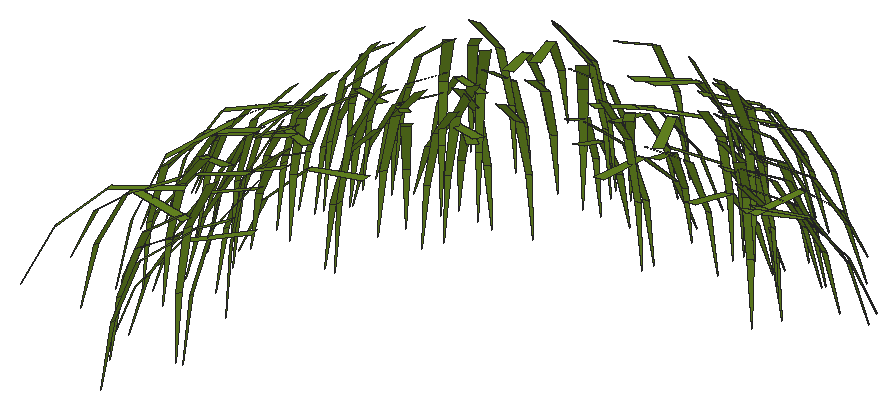
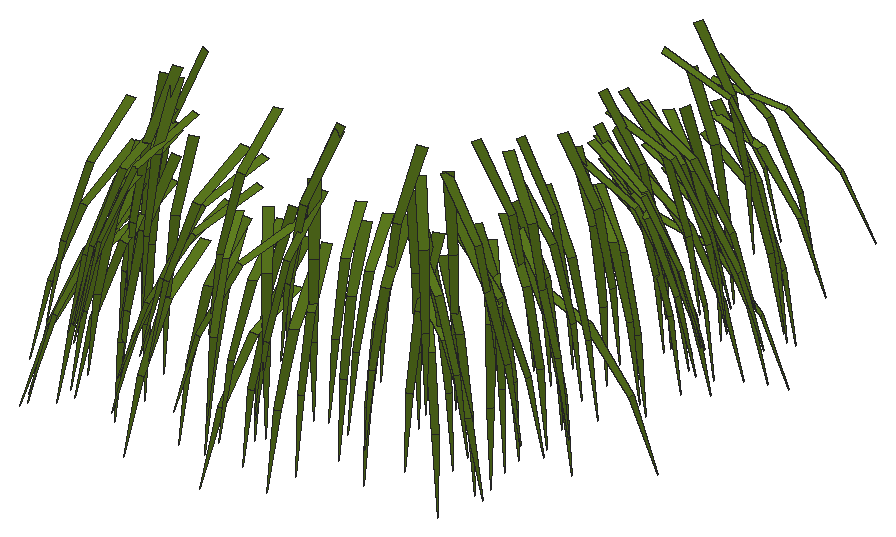
# SketchUp Ruby script. Lengths in inches.
U = 1.inch
M = Sketchup.active_model
def pt(a) = Geom::Point3d.new(a.map { |v| v * U })
def face(e, loops, mat)
  f = e.add_face(loops[0].map { |a| pt(a) })
  loops[1..].each { |l| e.add_face(l.map { |a| pt(a) }).erase! }
  f.material = f.back_material = mat if mat
  f
end
# faces: each face lists its corners as indices into pts; further lists are holes
def faces(e, pts, list, mat = nil) = list.each { |f| face(e, (f[0].is_a?(Array) ? f : [f]).map { |l| l.map { |i| pts[i] } }, mat) }
# xy, xz, yz: faces in a plane at the given z, y or x. An outline is a flat list of corners, or four numbers for a rectangle; further outlines are holes
def ring(l) = l.size == 4 ? [[l[0], l[1]], [l[2], l[1]], [l[2], l[3]], [l[0], l[3]]] : l.each_slice(2).to_a
def flat(e, list, mat, &to3) = list.each { |f| face(e, (f[0].is_a?(Array) ? f : [f]).map { |l| ring(l).map { |u, v| to3.(u, v) } }, mat) }
def xy(e, z, list, mat = nil) = flat(e, list, mat) { |x, y| [x, y, z] }
def xz(e, y, list, mat = nil) = flat(e, list, mat) { |x, z| [x, y, z] }
def yz(e, x, list, mat = nil) = flat(e, list, mat) { |y, z| [x, y, z] }
def lines(e, pts, list) = list.each { |a, b| e.add_line(pt(pts[a]), pt(pts[b])) }
# prism: a flat outline (further loops are holes) pulled along v
def prism(e, loops, v, mat = nil)
  f = face(e, loops, mat); d = Geom::Vector3d.new(v.map { |x| x * U })
  f.pushpull(f.normal.samedirection?(d) ? d.length : -d.length)
end
def box(e, o, s, mat = nil) = prism(e, [[o, [o[0] + s[0], o[1], o[2]], [o[0] + s[0], o[1] + s[1], o[2]], [o[0], o[1] + s[1], o[2]]]], [0, 0, s[2]], mat)
def at(x, y, z, deg = 0) = Geom::Transformation.translation(pt([x, y, z])) * Geom::Transformation.rotation(ORIGIN, Z_AXIS, deg.degrees)
def axes(o, x, y, z) = Geom::Transformation.new([*x, 0, *y, 0, *z, 0, *pt(o).to_a, 1])
def part(name) = M.definitions.add(name)
# library, detail: a bought-in or finely detailed component or shape, given as its bounding box
def library(name, o, s) = part(name).tap { |d| box(d.entities, o, s) }
def detail(e, o, s) = box(e.add_group.entities, o, s)
def put(e, d, t, mat = nil) = e.add_instance(d, t).tap { |i| i.material = mat if mat }
def group(e, t, mat = nil) = e.add_group.tap { |g| g.transformation = t; g.material = mat if mat }.entities
root = M.entities
M.materials.add("[0061_OliveDrab]").color = [107, 142, 35]
p = [[547.6,21.32,549.34],[547.56,21.51,549.34],[547.28,21.36,546.73],[547.37,28.64,549.33],[547.44,28.8125,549.33],[546.91,28.93,546.76],
  [548.89,31.45,549.33],[548.99,31.6,549.33],[548.51,31.82,546.76],[560.32,34.67,549.36],[560.5,34.73,549.36],[560.25,35.21,546.79],
  [546.9,18.21,549.5],[546.87,18.44,549.5],[546.46,18.28,546.91],[545.88,20.63,549.3125],[545.83,20.82,549.3125],[544.94,20.49,546.86],
  [548.84,33.23,549.46],[548.99,33.375,549.46],[548.21,34.05,547.05],[560.09,33.66,549.64],[560.29,33.77,549.64],[560.08,33.92,547.03],
  [555.03,34.76,549.55],[555.24,34.77,549.55],[555.11,35.23,546.97],[558.47,35.98,549.375],[558.68,36.02,549.375],[558.39,37.07,546.98],
  [545.65,27.41,549.44],[545.67,27.625,549.44],[544.48,27.64,547.1],[551.32,33.5,549.6875],[551.51,33.57,549.6875],[551.25,33.95,547.1],
  [562.55,35.57,549.5625],[562.74,35.53,549.5625],[562.83,36.35,547.07],[546.13,20.92,549.68],[546.16,21.11,549.68],[545.27,21.13,547.21],
  [548.18,31.25,549.77],[548.35,31.39,549.77],[547.83,31.85,547.24],[557.26,35.12,549.75],[557.48,35.13,549.75],[557.32,35.67,547.18],
  [553.46,35.38,549.62],[553.67,35.45,549.62],[553.23,36.33,547.18],[562.35,35.82,549.6],[562.54,35.77,549.6],[562.73,36.85,547.21],
  [555,36.3,549.5625],[555.22,36.32,549.5625],[554.97,37.54,547.25],[549.66,31.51,549.93],[549.78,31.7,549.93],[549.43,31.78,547.33],
  [555.36,33.95,549.95],[555.56,33.98,549.95],[555.43,34.2,547.34],[561.75,35.34,549.78],[561.95,35.32,549.78],[561.92,36.05,547.26],
  [546.66,18.8,550.07],[546.73,18.97,550.07],[546.16,19.1,547.51],[548,20.1,550.12],[548.07,20.31,550.12],[547.86,20.26,547.5],
  [548.34,27.75,550.12],[548.36,27.96,550.12],[548.18,27.86,547.5],[550.37,32.6,550.1],[550.58,32.68,550.1],[550.33,33.06,547.52],
  [548.21,30.1,550.19],[548.3125,30.3,550.19],[547.88,30.39,547.6],[556.09,35.37,550.07],[556.27,35.46,550.07],[555.81,36.22,547.6],
  [548.1,32.47,549.99],[548.21,32.67,549.99],[547.11,33.17,547.66],[552.88,34.93,550.2],[553.05,35.01,550.2],[552.64,35.65,547.6875],
  [546.86,23.9375,550.36],[546.91,24.12,550.36],[546.35,24.15,547.79],[560.23,34.5,550.43],[560.44,34.51,550.43],[560.32,34.91,547.84],
  [560.85,35.47,550.33],[561.07,35.45,550.33],[561.04,36.24,547.82],[559.19,35.45,550.33],[559.375,35.4,550.33],[559.49,36.29,547.86],
  [545.93,22.43,550.5],[545.95,22.625,550.5],[545.05,22.65,548.04],[546.07,23.74,550.53],[546.1,23.96,550.53],[545.32,23.95,548.02],
  [561.21,35.4,550.5],[561.41,35.41,550.5],[561.27,36.15,547.98],[546.59,19.18,550.625],[546.67,19.39,550.625],[545.9,19.57,548.12],
  [547.7,31.3,550.62],[547.84,31.43,550.62],[547.17,32,548.14],[548.21,22.54,550.78],[548.16,22.73,550.78],[548.02,22.6,548.16],
  [546.58,25.91,550.64],[546.7,26.1,550.64],[545.9,26.48,548.17],[547.51,30.27,550.71],[547.5625,30.46,550.71],[546.74,30.58,548.21],
  [547.32,29.86,550.89],[547.43,30.03,550.89],[546.82,30.29,548.34],[550.74,31.72,551.06],[550.88,31.86,551.06],[550.67,31.93,548.44],
  [551.68,34.29,550.9],[551.87,34.39,550.9],[551.45,34.98,548.375],[561.55,36.47,550.69],[561.74,36.47,550.69],[561.61,37.81,548.4375],
  [561.05,33.64,551.18],[561.24,33.6,551.18],[561.1875,33.81,548.56],[554.27,34.91,551.1],[554.4375,35.04,551.1],[553.8,35.7,548.64],
  [562.6,35.41,551.08],[562.8,35.375,551.08],[562.84,36.22,548.59],[555.01,35.76,551.05],[555.21,35.82,551.05],[554.83,36.76,548.62],
  [550.99,33.71,551.21],[551.21,33.78,551.21],[550.9,34.34,548.66],[558.8125,34.22,551.34],[559,34.29,551.34],[558.79,34.58,548.74],
  [560.8,35.24,551.18],[561,35.3,551.18],[560.68,36.02,548.67],[546.84,28.06,551.31],[546.9375,28.23,551.31],[546.22,28.51,548.79],
  [553.33,33.7,551.4],[553.51,33.84,551.4],[553.17,34.08,548.81],[546.39,24.22,551.49],[546.43,24.43,551.49],[545.82,24.43,548.9375],
  [547.5625,26.37,551.49],[547.6875,26.56,551.49],[547.31,26.67,548.89],[550.07,30.69,551.52],[550.21,30.83,551.52],[550.02,30.88,548.9],
  [547.75,30.94,551.375],[547.85,31.15,551.375],[546.97,31.42,548.91],[556.42,35.71,551.41],[556.63,35.65,551.41],[556.79,36.55,548.94],
  [545.75,21.83,551.43],[545.77,22.05,551.43],[544.73,22.04,549.02],[547.44,23.9375,551.61],[547.46,24.15,551.61],[547.125,24.08,549],
  [546.24,26.71,551.5625],[546.35,26.875,551.5625],[545.46,27.35,549.14],[547.48,28.04,551.6875],[547.52,28.24,551.6875],[547.08,28.22,549.1],
  [546.59,29.89,551.56],[546.6875,30.05,551.56],[545.8125,30.48,549.125],[554.3,34.92,551.6],[554.49,34.9375,551.6],[554.33,35.5625,549.06],
  [547.46,20.26,551.78],[547.5625,20.45,551.78],[547.14,20.54,549.1875],[548.38,32.75,551.55],[548.49,32.91,551.55],[547.5,33.45,549.18],
  [547.48,21,551.36],[547.41,21.26,551.36],[548.3,21.41,551.87],[548.25,21.68,551.87],[546.69,24.09,551.82],[546.63,24.29,551.82],
  [546.04,24.01,549.27],[545.98,24.67,551.7],[546.03,24.86,551.7],[545.07,25.02,549.26],[548.32,28.2,551.74],[548.42,28.44,551.74],
  [549.72,30.83,551.74],[549.87,31.04,551.74],[555.6875,35.79,551.66],[555.87,35.89,551.66],[555.1875,36.9,549.34],[547.51,25.99,552.04],
  [547.5625,26.2,552.04],[547.2,26.18,549.44],[547.5,27.18,551.28],[547.54,27.48,551.28],[560.59,33.65,551.77],[560.84,33.73,551.77],
  [558.73,34.25,551.33],[559.03,34.3,551.33],[561.19,35.1,551.95],[561.4,35.04,551.95],[561.47,35.73,549.41],[547.86,18.27,551.94],
  [547.82,18.59,551.94],[549.98,31.97,551.46],[550.19,32.17,551.46],[558.5,35.71,551.85],[558.68,35.64,551.85],[558.97,36.68,549.45],
  [560.34,33.11,552.2],[560.62,33.26,552.2],[555.03,33.75,551.98],[555.33,33.77,551.98],[553.96,33.85,551.69],[554.26,33.96,551.69],
  [561.87,34.18,551.59],[562.15,34.11,551.59],[562.18,34.14,551.74],[562.44,34.08,551.74],[555.17,34.36,551.33],[555.48,34.4,551.33],
  [546.45,17.94,552.27],[546.46,18.15,552.27],[545.81,18.09,549.73],[547.59,20.7,551.85],[547.625,20.97,551.85],[548.13,27.53,552.33],
  [548.17,27.7,552.33],[547.89,27.67,549.72],[548.58,30.61,552.29],[548.66,30.79,552.29],[548.1875,30.87,549.71],[551.65,32.57,552.125],
  [551.91,32.67,552.125],[557.3125,33.97,552.11],[557.625,34,552.11],[548.96,30.2,552.05],[549.2,30.4,552.05],[561.59,34.02,552.05],
  [561.875,34,552.05],[546.2,22.5,552.28],[546.3125,22.6875,552.28],[545.34,23.14,549.88],[547.67,23.49,552.53],[547.69,23.6875,552.53],
  [547.37,23.625,549.93],[550.29,31.0625,552.44],[550.46,31.33,552.44],[560.59,33.16,552.49],[560.8,33.23,552.49],[560.625,33.39,549.87],
  [549.6875,31.5,551.84],[549.85,31.78,551.84],[549.71,32.625,552.51],[549.87,32.77,552.51],[549.39,33.15,549.96],[555.42,33.33,552.5],
  [555.69,33.375,552.5],[550.83,34.73,552.36],[551.02,34.82,552.36],[550.49,35.72,549.95],[561.19,35.39,552.49],[561.41,35.35,552.49],
  [561.42,36.11,549.97],[547.75,18.34,552.41],[547.84,18.58,552.41],[548.48,19.9,552.7],[548.58,20.19,552.7],[548.82,27.67,552.7],
  [548.84,27.97,552.7],[548.66,28.85,552.67],[548.7,29.04,552.67],[548.375,29.01,550.07],[550.65,31.7,552.55],[550.9375,31.8,552.55],
  [556.7,33.94,552.18],[556.96,34.0625,552.18],[545.27,19.38,552.45],[545.32,19.57,552.45],[544.02,19.8,550.17],[546.21,22.79,552.67],
  [546.28,22.99,552.67],[545.34,23.22,550.23],[546.9,22.94,552.76],[546.95,23.15,552.76],[546.42,23.15,550.1875],[547.61,29.26,552.79],
  [547.72,29.44,552.79],[547.19,29.63,550.22],[549.02,29.64,552.65],[549.16,29.93,552.65],[551.55,32.36,552.77],[551.75,32.41,552.77],
  [551.57,32.72,550.17],[554.84,32.98,552.83],[555.06,32.96,552.83],[554.97,33.2,550.21],[554.68,33.38,552.85],[554.88,33.375,552.85],
  [554.79,33.68,550.24],[553.46,33.65,552.42],[553.7,33.77,552.42],[558.81,34.03,552.51],[559.06,33.97,552.51],[560.66,34.09,552.55],
  [560.97,34.05,552.55],[551.37,35.08,552.78],[551.55,35.17,552.78],[551.01,35.99,550.35],[562.01,35.45,552.75],[562.2,35.46,552.75],
  [562.03,36.375,550.29],[547.65,19.08,552.98],[547.71,19.26,552.98],[547.32,19.29,550.39],[545.89,22.03,552.87],[545.9,22.25,552.87],
  [544.9,22.2,550.44],[547.9,23.65,552.75],[547.96,23.91,552.75],[545.86,24.75,552.8],[545.91,24.93,552.8],[544.82,25.1,550.42],
  [545.76,24.79,552.77],[545.79,24.97,552.77],[544.67,25.0625,550.39],[560.24,33.62,552.9],[560.53,33.63,552.9],[547.46,22.17,552.62],
  [547.5,22.44,552.62],[547.49,23.51,552.72],[547.53,23.82,552.72],[559.83,34,553.0625],[560.02,34.06,553.0625],[559.79,34.42,550.47],
  [561.24,34.05,552.75],[561.52,34.0625,552.75],[560.78,35.23,553.03],[560.96,35.18,553.03],[561.06,35.89,550.51],[560.89,35.44,552.96],
  [561.09,35.43,552.96],[561.05,36.27,550.48],[557.9,35.66,552.92],[558.11,35.61,552.92],[558.23,36.5,550.45],[557.68,35.7,552.93],
  [557.9,35.7,552.93],[557.79,36.58,550.46],[545.57,16.99,553],[545.52,17.17,553],[544.42,16.77,550.65],[547.4,18.6,553.18],
  [547.3,18.8,553.18],[546.9,18.47,550.6],[547.82,18.66,552.89],[547.93,18.95,552.89],[546.16,22.8,553.14],[546.14,23,553.14],
  [545.4,22.85,550.625],[547.8125,25.07,552.8],[547.98,25.34,552.8],[548.74,30.16,552.74],[548.93,30.35,552.74],[560.5625,33.78,553.16],
  [560.78,33.8,553.16],[560.63,34.14,550.56],[548.88,29.87,552.91],[548.95,30.13,552.91],[560.86,32.22,553.27],[561.04,32.14,553.27],
  [561.01,32.33,550.65],[561.58,34.43,552.35],[561.83,34.4375,552.35],[548.67,22.62,553.36],[548.61,22.875,553.36],[548.36,29.17,553.2],
  [548.5,29.41,553.2],[552.22,33.125,553.1875],[552.49,33.26,553.1875],[555.42,34.14,553.07],[555.7,34.22,553.07],[551.09,31.31,553.63],
  [551.29,31.5,553.63],[555.2,33.64,553.2],[555.44,33.82,553.2],[562.33,34.01,553.29],[562.62,33.97,553.29],[551.34,32.54,553.53],
  [551.64,32.64,553.53],[560.9,33.13,553.75],[561.17,33.08,553.75],[561.13,33.91,553.41],[561.41,33.99,553.41],[550.03,26.88,551.92],
  [550.07,27.25,551.92],[547.99,27.38,553.57],[548.12,27.625,553.57],[555.43,31.79,551.8],[555.81,31.84,551.8],[559.12,31.8,552.18],
  [559.49,31.86,552.18],[559.06,33.42,553.83],[559.33,33.53,553.83],[549.88,21.58,552.25],[549.8,21.9,552.25],[547.41,21.63,553.46],
  [547.44,21.93,553.46],[549.08,30.29,553.55],[549.21,30.57,553.55],[553.85,32.97,553.87],[554.09,33.17,553.87],[555.92,34.18,553.48],
  [556.21,34.09,553.48],[556.33,34.71,553.93],[556.52,34.74,553.93],[556.34,35.36,551.39],[556.33,35.08,552.49],[547.59,23.97,553.8125],
  [547.64,24.27,553.8125],[548.27,25.85,553.96],[548.44,26.11,553.96],[551.66,30.15,552.34],[551.92,30.4,552.34],[550.38,30.33,554.1],
  [550.58,30.53,554.1],[548.22,23.82,554.11],[548.25,24.12,554.11],[547.65,25.71,553.53],[547.8125,25.94,553.53],[548,28.97,553.57],
  [548.14,29.1875,553.57],[549.87,31.72,553.45],[550.02,31.95,553.45],[561.22,31.875,552.66],[561.5625,31.78,552.66],[554.4,33.71,553.93],
  [554.66,33.73,553.93],[547.51,24.2,553.78],[547.58,24.46,553.78],[550.09,27.43,553.52],[550.22,27.73,553.52],[548.39,27.83,554.14],
  [548.44,28.11,554.14],[551.28,29.72,553.54],[551.46,29.98,553.54],[554.74,31.61,552.8125],[555.11,31.74,552.8125],[561.62,31.87,552.91],
  [561.9375,31.79,552.91],[556.6,34.04,553.4],[556.85,34.18,553.4],[548.26,19.81,554.24],[548.4,20.09,554.24],[547.88,24.38,554.14],
  [547.8,24.67,554.14],[551.85,30.21,552.58],[552.05,30.55,552.58],[561.125,31.78,553.53],[561.43,31.875,553.53],[557.86,34.13,553.85],
  [558.12,34.03,553.85],[549.86,18.45,553.63],[549.82,18.84,553.63],[549.82,20.38,553.21],[549.86,20.72,553.21],[549.87,21.68,553.96],
  [549.81,22.01,553.96],[560.84,33.88,554.25],[561.13,33.8,554.25],[548.28,25.74,554.54],[548.36,26.05,554.54],[555.09,31.74,553.66],
  [555.45,31.75,553.66],[550.35,28.43,553.4],[550.65,28.67,553.4],[552.36,30.7,553.83],[552.68,30.83,553.83],[557.46,31.8125,553.59],
  [557.84,31.84,553.59],[561.36,31.84,553.5],[561.71,31.8125,553.5],[561.04,31.74,554.32],[561.38,31.92,554.32],[557.67,31.76,553.26],
  [557.99,31.9,553.26],[547.72,17.82,554.57],[547.73,18.12,554.57],[547.65,21.57,554.26],[547.8125,21.84,554.26],[548.79,27.34,554.87],
  [548.84,27.6,554.87],[549.52,30.18,554.7],[549.625,30.44,554.7],[561.62,31.82,552.66],[561.9375,31.83,552.66],[549.78,17.52,553.86],
  [549.89,17.82,553.86],[547.26,18.84,554.07],[547.33,19.11,554.07],[551.72,30.13,554.44],[551.92,30.46,554.44],[554.45,31.54,553.625],
  [554.74,31.68,553.625],[551.52,33.125,554.32],[551.79,33.25,554.32],[548.42,23.35,555.05],[548.46,23.63,555.05],[547.77,23.47,552.87],
  [550.48,31.68,554.84],[550.71,31.88,554.84],[555.62,31.8,554.625],[555.96,31.85,554.625],[558.25,31.87,553.88],[558.5625,31.79,553.88],
  [560.39,31.85,553.89],[560.77,31.81,553.89],[560.86,32.67,555.05],[561.02,32.72,555.05],[560.73,32.62,555.05],[560.92,34.02,554.71],
  [561.22,33.97,554.71],[549.8125,21.8,553.72],[549.86,22.14,553.72],[550.68,28.77,554.48],[550.85,29.12,554.48],[551.26,29.89,554.35],
  [551.62,30.01,554.35],[549.78,19.45,554.93],[549.89,19.8,554.93],[547.69,22.22,554.76],[547.79,22.5,554.76],[549.8125,23.17,553.9],
  [549.86,23.55,553.9],[550.17,27.55,554.95],[550.2,27.91,554.95],[550.36,28.41,553.83],[550.61,28.64,553.83],[549.4,28.65,555.18],
  [549.46,28.92,555.18],[561.33,31.82,554.14],[561.67,31.84,554.14],[562.1,33.93,554.89],[562.37,33.95,554.89],[547.97,22.68,555.15],
  [548.03,22.96,555.15],[549.8,23.17,554.5],[549.875,23.48,554.5],[549.73,23.81,554.07],[549.94,24.13,554.07],[547.53,24.3,554.77],
  [547.6,24.56,554.77],[547.47,24.46,554.72],[547.52,24.72,554.72],[548.5625,28.64,555.15],[548.72,28.9,555.15],[551.68,31.56,555.26],
  [551.97,31.62,555.26],[551.86,32.03,553.97],[554.72,32.375,555.38],[555.03,32.34,555.38],[552.14,33.54,554.77],[552.39,33.67,554.77],
  [549.77,17.87,554.46],[549.91,18.22,554.46],[547.53,21.88,554.91],[547.55,22.2,554.91],[551.04,29.26,554.27],[551.125,29.58,554.27],
  [560.3,31.82,554.82],[560.66,31.84,554.82],[554.6,32.65,555.37],[554.89,32.63,555.37],[557.46,34.13,555.01],[557.76,34.05,555.01],
  [557.64,34.13,555.04],[557.96,34.13,555.04],[547.4,17.46,554.83],[547.33,17.71,554.83],[548.49,18.76,555.45],[548.58,19.01,555.45],
  [560.375,33.91,555.27],[560.64,33.84,555.27],[560.75,33.97,555.13],[561.04,33.95,555.13],[547.61,22.85,555.32],[547.59,23.14,555.32],
  [556.05,31.78,554.02],[556.4,31.88,554.02],[560.08,33.11,555.52],[560.35,33.2,555.52],[548.39,19.06,555.57],[548.26,19.33,555.57],
  [550.18,28,554.69],[550.36,28.29,554.69],[553.14,31.21,554.73],[553.48,31.38,554.73],[556.65,31.71,554.25],[556.94,31.94,554.25],
  [560.61,32.94,555.65],[560.92,32.98,555.65],[560.63,31.84,555.86],[560.89,31.72,555.86],[561.95,31.86,554.73],[562.31,31.8,554.73],
  [549.9375,22.9,555.64],[549.86,23.22,555.64],[557.83,31.74,553.6875],[558.14,31.91,553.6875],[561.7,31.78,554.84],[562.05,31.88,554.84],
  [549.82,21.36,554.47],[549.86,21.73,554.47],[549.74,24.27,554.21],[549.93,24.55,554.21],[551.06,29.34,554.97],[551.23,29.6875,554.97],
  [551.95,30.3,554.19],[552.14,30.6,554.19],[552,30.48,555.02],[552.37,30.6,555.02],[555.17,31.82,554.34],[555.53,31.71,554.34],
  [549.85,26.32,555.08],[550.02,26.62,555.08],[550.11,27.625,554.38],[550.27,27.89,554.38],[552.08,30.27,555.83],[552.32,30.51,555.83],
  [560.57,31.74,555.95],[560.87,31.68,555.95],[560.9,31.67,555.95],[549.79,23.53,554.89],[549.88,23.85,554.89],[549.81,23.56,555.16],
  [549.87,23.92,555.16],[559.67,31.69,555.71],[560,31.81,555.71],[556.98,31.89,554.89],[557.3,31.77,554.89],[554.96,31.5,555.74],
  [555.26,31.74,555.74],[554.59,31.59,555.47],[554.91,31.625,555.47],[556.47,33.42,556.22],[556.75,33.46,556.22],[549.82,24.78,555.79],
  [550.04,25.11,555.79],[549.8,18.17,554.19],[549.88,18.5,554.19],[549.96,23.62,556.06],[550,23.99,556.06],[549.95,24.93,555.66],
  [549.85,25.29,555.66],[550.27,27.44,555.93],[550.34,27.79,555.93],[551.34,29.35,556.34],[551.58,29.6,556.34],[549.9,18.94,556.09],
  [550.07,19.28,556.09],[560.27,31.79,555.74],[560.63,31.7,555.74],[549.74,20.29,555.2],[549.94,20.61,555.2],[552.55,30.82,555.04],
  [552.875,30.97,555.04],[550.01,25.26,556.45],[550.11,25.64,556.45],[549.95,17.64,555.94],[549.97,18.01,555.94],[548.59,18.07,555.09],
  [549.88,24.02,555.68],[549.93,24.34,555.68],[551.43,29.38,556.32],[551.56,29.7,556.32],[560.51,31.74,555.94],[560.87,31.68,555.94],
  [560.88,31.68,555.94],[549.88,18.11,555.35],[549.8,18.42,555.35],[549.9,21.4,555.93],[550.02,21.75,555.93],[549.89,23.69,555.77],
  [549.96,24.01,555.77],[551.9,30.01,556.28],[552.18,30.25,556.28],[553.29,31.27,555.42],[553.6,31.4375,555.42],[549.95,21.7,555.93],
  [549.97,22.09,555.93],[550.4,26.96,556.9],[550.47,27.27,556.9],[562.26,31.65,556.17],[562.59,31.67,556.17],[550.17,23.09,556.98],
  [550.22,23.4375,556.98],[556.82,31.76,555.93],[557.1875,31.66,555.93],[557.61,31.69,556.01],[558,31.69,556.01],[550.06,22.2,556.66],
  [550.14,22.55,556.66],[550.39,27.5,556.65],[550.58,27.82,556.65],[561.17,31.24,557.24],[561.52,31.36,557.24],[560.57,31.64,556.33],
  [560.91,31.62,556.33],[551.13,28.25,557.12],[551.2,28.59,557.12],[550.04,22.99,556.3],[550.02,23.35,556.3],[552.05,29.76,557.14],
  [552.41,29.84,557.14],[559.73,31.65,556.44],[560.05,31.56,556.44],[550.31,18.12,557.23],[550.41,18.4375,557.23],[554.52,30.83,557.49],
  [554.89,30.78,557.49],[554.5,30.92,557.34],[554.86,30.91,557.34],[560.68,31.23,557.26],[561.01,31.35,557.26],[550.33,20,557.0625],
  [550.16,20.34,557.0625],[560.8,31.1,557.51],[561.17,31.14,557.51],[560.08,30.75,558.18],[560.4,30.6,558.18],[556.77,31.13,557.46],
  [557.1,31.18,557.46]]
faces(root,p,[[0,1,2],[3,4,5],[6,7,8],[9,10,11],[12,13,14],[15,16,17],[18,19,20],[21,22,23],
  [24,25,26],[27,28,29],[30,31,32],[33,34,35],[36,37,38],[39,40,41],[42,43,44],[45,46,47],
  [48,49,50],[51,52,53],[54,55,56],[57,58,59],[60,61,62],[63,64,65],[66,67,68],[69,70,71],
  [72,73,74],[75,76,77],[78,79,80],[81,82,83],[84,85,86],[87,88,89],[90,91,92],[93,94,95],
  [96,97,98],[99,100,101],[102,103,104],[105,106,107],[108,109,110],[111,112,113],[114,115,116],[117,118,119],
  [120,121,122],[123,124,125],[126,127,128],[129,130,131],[132,133,134],[135,136,137],[138,139,140],[141,142,143],
  [144,145,146],[147,148,149],[150,151,152],[153,154,155],[156,157,158],[159,160,161],[162,163,164],[165,166,167],
  [168,169,170],[171,172,173],[174,175,176],[177,178,179],[180,181,182],[183,184,185],[186,187,188],[189,190,191],
  [192,193,194],[195,196,197],[198,199,200],[201,202,203],[204,205,16,15],[206,207,1,0],[208,209,210],[211,212,213],
  [214,215,4,3],[216,217,7,6],[218,219,220],[221,222,223],[224,225,31,30],[226,227,10,9],[228,229,28,27],[230,231,232],
  [233,234,13,12],[235,236,19,18],[237,238,239],[240,241,22,21],[242,243,25,24],[244,245,49,48],[246,247,52,51],[248,249,37,36],
  [250,251,55,54],[252,253,254],[255,256,40,39],[257,258,259],[260,261,262],[263,264,34,33],[265,266,46,45],[267,268,43,42],
  [269,270,64,63],[271,272,273],[274,275,276],[277,278,58,57],[279,280,281],[282,283,85,84],[284,285,286],[287,288,61,60],
  [289,290,291],[292,293,294],[295,296,67,66],[297,298,70,69],[299,300,73,72],[301,302,303],[304,305,76,75],[306,307,82,81],
  [308,309,310],[311,312,313],[314,315,316],[317,318,319],[320,321,79,78],[322,323,324],[325,326,327],[328,329,330],
  [331,332,88,87],[333,334,100,99],[335,336,97,96],[337,338,339],[340,341,342],[343,344,345],[346,347,348],[349,350,91,90],
  [351,352,353],[354,355,356],[357,358,94,93],[359,360,103,102],[361,362,106,105],[363,364,365],[366,367,109,108],[368,369,370],
  [371,372,373],[374,375,376],[377,378,379],[380,381,382],[383,384,385],[386,387,112,111],[388,389,390],[391,392,121,120],
  [393,394,115,114],[395,396,397],[398,399,124,123],[400,401,402],[403,404,136,135],[405,406,118,117],[407,408,127,126],[409,410,133,132],
  [411,412,148,147],[413,414,130,129],[415,416,142,141],[417,418,145,144],[419,420,151,150],[421,422,139,138],[423,424,157,156],[425,426,225,224],
  [427,428,160,159],[429,430,251,250],[431,432,229,228],[433,434,154,153],[435,436,205,204],[437,438,181,180],[439,440,175,174],[441,442,163,162],
  [443,444,178,177],[445,446,447,448],[449,450,166,165],[451,452,169,168],[453,454,236,235],[455,456,172,171],[457,458,184,183],[459,460,187,186],
  [461,462,193,192],[463,464,202,201],[465,466,247,246],[467,468,196,195],[469,470,212,211],[471,472,215,214],[473,474,190,189],[475,476,217,216],
  [477,478,245,244],[479,480,249,248],[481,482,448,219,218],[483,484,199,198],[485,486,209,208],[487,488,283,282],[489,490,227,226],[491,492,238,237],
  [493,494,234,233],[495,496,256,255],[497,498,207,206],[499,500,231,230],[501,502,222,221],[503,504,243,242],[505,506,268,267],[507,508,264,263],
  [509,510,266,265],[511,512,270,269],[513,514,241,240],[515,516,307,306],[517,518,253,252],[519,520,272,271],[521,522,258,257],[523,524,261,260],
  [525,526,404,403],[527,528,296,295],[529,530,309,308],[531,532,278,277],[533,534,332,331],[535,536,290,289],[537,538,275,274,539],[540,541,285,284],
  [542,543,288,287],[544,545,334,333],[546,547,336,335],[548,549,280,279,550],[551,552,293,292],[553,554,360,359],[555,556,321,320],[557,558,305,304],
  [559,560,298,297],[561,562,312,311],[563,564,362,361,539],[565,566,300,299],[567,568,394,393],[569,570,302,301],[571,572,367,366],[573,574,341,340],
  [575,576,315,314],[577,578,350,349],[579,580,392,391],[581,582,352,351],[583,584,355,354],[585,586,318,317],[587,588,589,323,322],[590,591,326,325],
  [592,593,338,337],[594,595,387,386],[596,597,347,346],[598,599,399,398],[600,601,358,357],[602,603,329,328],[604,605,375,374],[606,607,378,377],
  [608,609,381,380],[610,611,344,343],[612,613,369,368],[614,615,372,371],[616,617,389,388],[618,619,412,411],[620,621,364,363],[622,623,384,383],
  [624,625,408,407],[626,627,410,409],[628,629,416,415],[630,631,396,395],[632,633,401,400],[634,635,418,417],[636,637,406,405],[638,639,482,481],
  [640,641,424,423],[642,643,438,437],[644,645,460,459],[646,647,440,439],[648,649,464,463],[650,651,589,420,419],[652,653,444,443],[654,655,428,427],
  [656,657,462,461],[658,659,414,413],[660,661,662,422,421],[663,664,470,469],[665,666,450,449],[667,668,434,433],[669,670,492,491],[671,672,442,441],
  [673,674,468,467],[675,676,446,445],[677,678,452,451],[679,680,530,529],[681,682,458,457],[683,684,486,485],[685,686,474,473],[687,688,456,455],
  [689,690,484,483],[691,692,548,500,499],[693,694,520,519],[695,696,536,535],[697,698,502,501],[699,700,701,518,517],[702,703,584,583],[704,705,524,523],
  [706,707,708,552,551],[709,710,701,609,608],[711,712,562,561],[713,714,582,581],[715,716,541,540],[717,718,593,592],[719,720,597,596],[721,722,522,521],
  [723,724,574,573],[725,726,538,537],[727,728,605,604],[729,730,607,606],[731,732,576,575],[733,734,586,585],[735,736,549,548,550],[737,738,615,614],
  [739,740,570,569],[741,742,617,616],[743,744,588,587],[745,746,613,612],[747,748,611,610],[749,750,591,590],[751,752,603,602],[753,754,621,620],
  [755,756,623,622],[757,758,631,630],[759,760,661,707,633,632],[761,762,676,675]],"[0061_OliveDrab]")
